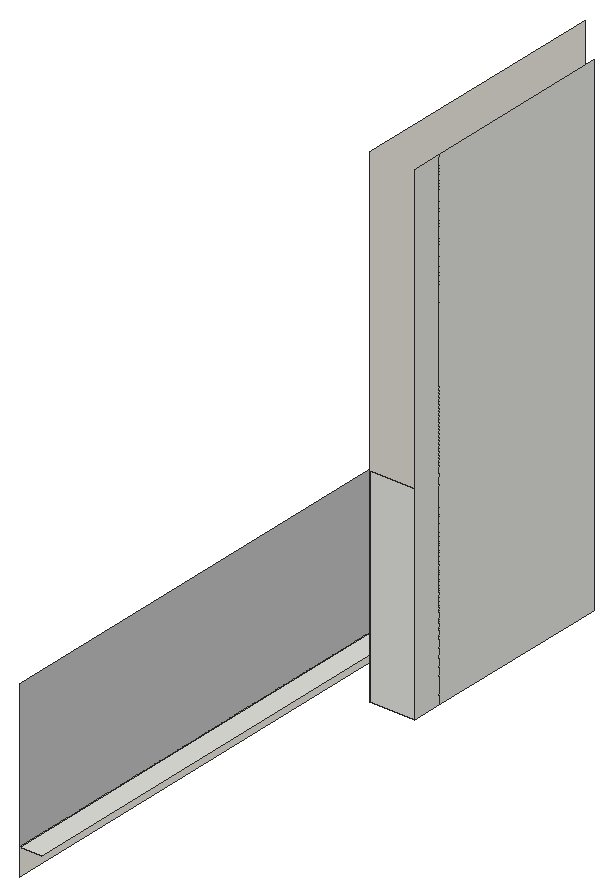
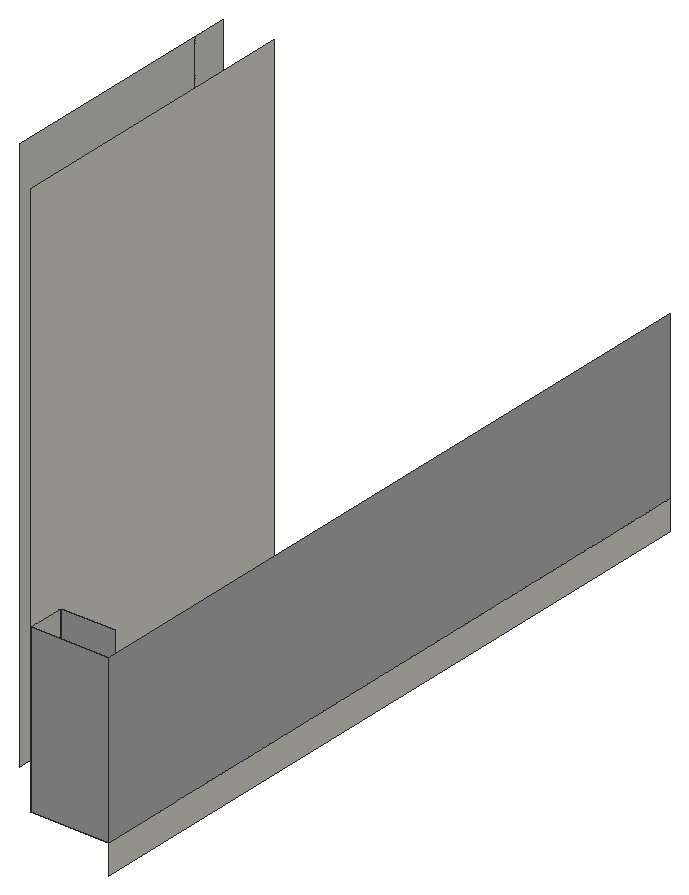
# SketchUp Ruby script. Lengths in inches.
U = 1.inch
M = Sketchup.active_model
def pt(a) = Geom::Point3d.new(a.map { |v| v * U })
def face(e, loops, mat)
  f = e.add_face(loops[0].map { |a| pt(a) })
  loops[1..].each { |l| e.add_face(l.map { |a| pt(a) }).erase! }
  f.material = f.back_material = mat if mat
  f
end
# faces: each face lists its corners as indices into pts; further lists are holes
def faces(e, pts, list, mat = nil) = list.each { |f| face(e, (f[0].is_a?(Array) ? f : [f]).map { |l| l.map { |i| pts[i] } }, mat) }
# xy, xz, yz: faces in a plane at the given z, y or x. An outline is a flat list of corners, or four numbers for a rectangle; further outlines are holes
def ring(l) = l.size == 4 ? [[l[0], l[1]], [l[2], l[1]], [l[2], l[3]], [l[0], l[3]]] : l.each_slice(2).to_a
def flat(e, list, mat, &to3) = list.each { |f| face(e, (f[0].is_a?(Array) ? f : [f]).map { |l| ring(l).map { |u, v| to3.(u, v) } }, mat) }
def xy(e, z, list, mat = nil) = flat(e, list, mat) { |x, y| [x, y, z] }
def xz(e, y, list, mat = nil) = flat(e, list, mat) { |x, z| [x, y, z] }
def yz(e, x, list, mat = nil) = flat(e, list, mat) { |y, z| [x, y, z] }
def lines(e, pts, list) = list.each { |a, b| e.add_line(pt(pts[a]), pt(pts[b])) }
# prism: a flat outline (further loops are holes) pulled along v
def prism(e, loops, v, mat = nil)
  f = face(e, loops, mat); d = Geom::Vector3d.new(v.map { |x| x * U })
  f.pushpull(f.normal.samedirection?(d) ? d.length : -d.length)
end
def box(e, o, s, mat = nil) = prism(e, [[o, [o[0] + s[0], o[1], o[2]], [o[0] + s[0], o[1] + s[1], o[2]], [o[0], o[1] + s[1], o[2]]]], [0, 0, s[2]], mat)
def at(x, y, z, deg = 0) = Geom::Transformation.translation(pt([x, y, z])) * Geom::Transformation.rotation(ORIGIN, Z_AXIS, deg.degrees)
def axes(o, x, y, z) = Geom::Transformation.new([*x, 0, *y, 0, *z, 0, *pt(o).to_a, 1])
def part(name) = M.definitions.add(name)
# library, detail: a bought-in or finely detailed component or shape, given as its bounding box
def library(name, o, s) = part(name).tap { |d| box(d.entities, o, s) }
def detail(e, o, s) = box(e.add_group.entities, o, s)
def put(e, d, t, mat = nil) = e.add_instance(d, t).tap { |i| i.material = mat if mat }
def group(e, t, mat = nil) = e.add_group.tap { |g| g.transformation = t; g.material = mat if mat }.entities
root = M.entities
M.materials.add("[Fencing Metal Straight]").color = [194, 195, 196]
M.materials.add("[Tile Limestone Large]").color = [237, 234, 224]
xy(root,17.625,[[0,0,0,413.49,46.1875,413.49,46.1875,390.99,14.48,390.99,14.48,0]])
xz(root,233.86,[[46.1875,17.625,76.4,155.84]])
xz(root,390.99,[[14.48,17.625,46.1875,115.1875]],"[Fencing Metal Straight]")
xz(root,413.49,[[0,17.625,46.1875,115.1875]],"[Fencing Metal Straight]")
yz(root,0,[[0,17.625,413.49,115.1875]],"[Fencing Metal Straight]")
yz(root,0,[[0,0,413.49,17.625]],"[Tile Limestone Large]")
yz(root,46.1875,[[390.99,17.625,413.49,115.1875]])
yz(root,46.1875,[[233.86,17.625,233.86,346.625,413.49,346.625,413.49,115.1875,390.99,115.1875,390.99,17.625]],"[Tile Limestone Large]")
yz(root,76.4,[[233.86,17.625,254.16,346.625],[254.16,17.625,383.27,346.625]])
